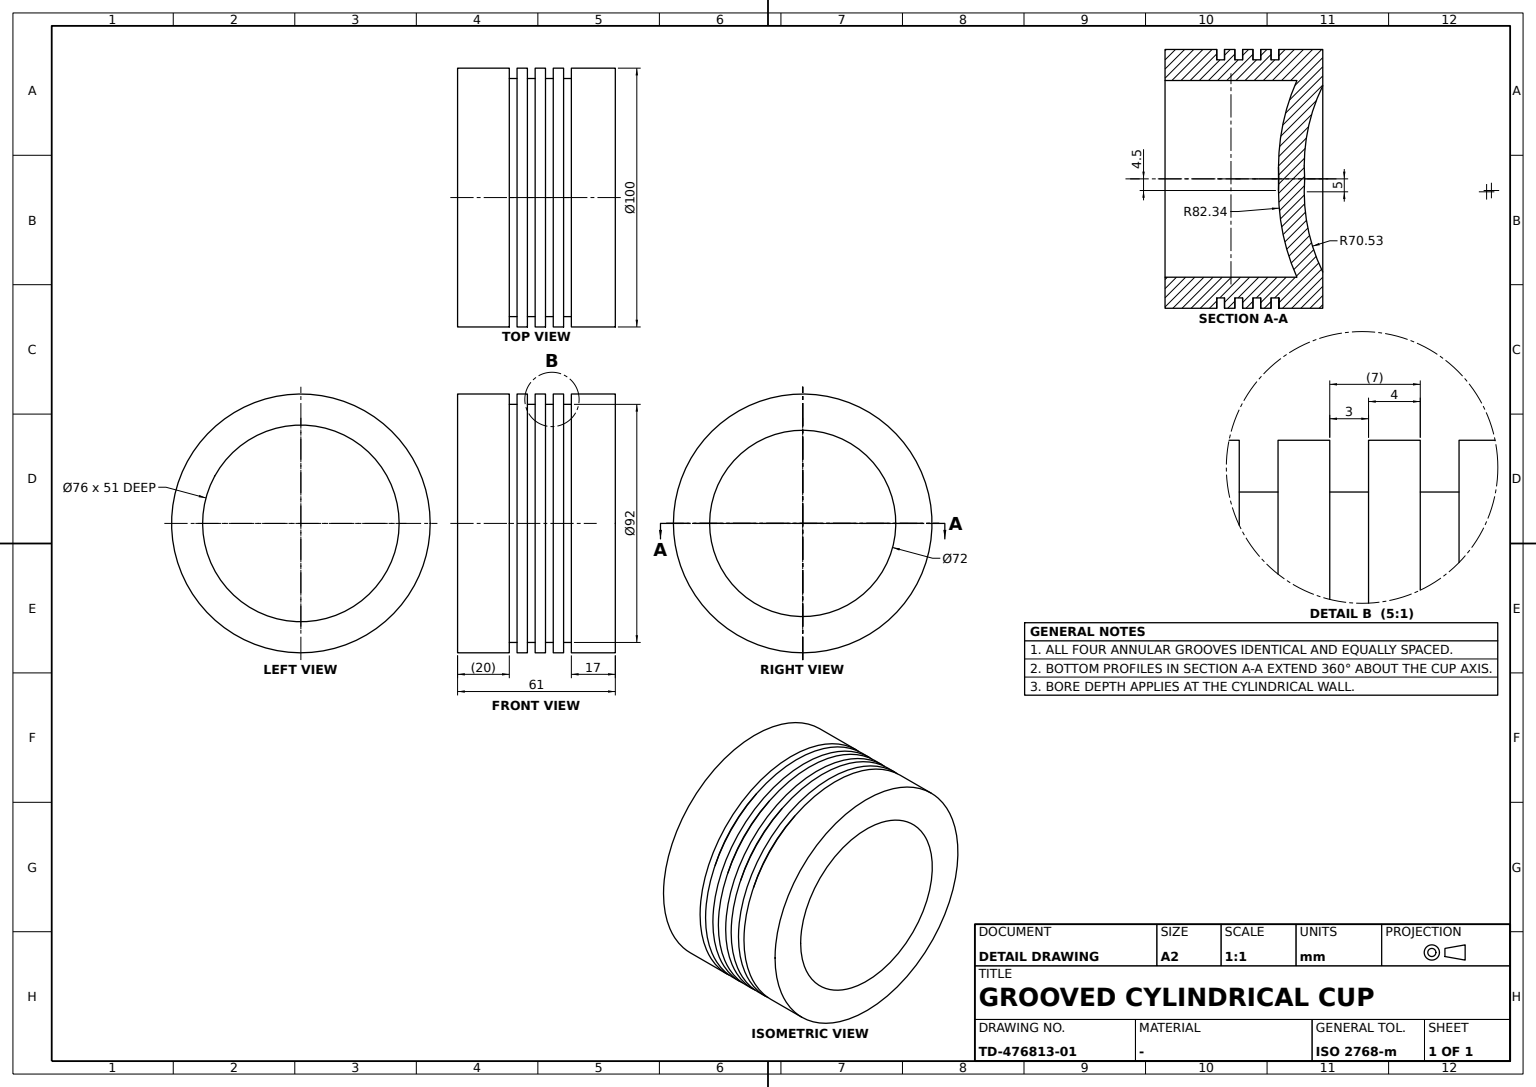
ISO-10303-21;
HEADER;
FILE_DESCRIPTION((''),'2;1');
FILE_NAME('','',(''),(''),'','','');
FILE_SCHEMA(('AUTOMOTIVE_DESIGN'));
ENDSEC;
DATA;
#1=APPLICATION_CONTEXT('');
#2=PRODUCT_CONTEXT('',#1,'mechanical');
#3=PRODUCT('','','',(#2));
#4=PRODUCT_DEFINITION_FORMATION('','',#3);
#5=PRODUCT_DEFINITION_CONTEXT('',#1,'design');
#6=PRODUCT_DEFINITION('','',#4,#5);
#7=PRODUCT_DEFINITION_SHAPE('','',#6);
#8=(LENGTH_UNIT()NAMED_UNIT(*)SI_UNIT(.MILLI.,.METRE.));
#9=(NAMED_UNIT(*)PLANE_ANGLE_UNIT()SI_UNIT($,.RADIAN.));
#10=(NAMED_UNIT(*)SI_UNIT($,.STERADIAN.)SOLID_ANGLE_UNIT());
#11=UNCERTAINTY_MEASURE_WITH_UNIT(LENGTH_MEASURE(1.E-05),#8,'distance_accuracy_value','');
#12=(GEOMETRIC_REPRESENTATION_CONTEXT(3)GLOBAL_UNCERTAINTY_ASSIGNED_CONTEXT((#11))GLOBAL_UNIT_ASSIGNED_CONTEXT((#8,#9,#10))REPRESENTATION_CONTEXT('',''));
#13=CARTESIAN_POINT('',(-40.368798,37.,22.053575));
#14=VERTEX_POINT('',#13);
#15=CARTESIAN_POINT('',(-40.368798,34.,22.053575));
#16=VERTEX_POINT('',#15);
#17=CARTESIAN_POINT('',(-40.368798,32.,22.053575));
#18=DIRECTION('',(0.,-1.,0.));
#19=VECTOR('',#18,1000.);
#20=LINE('',#17,#19);
#21=EDGE_CURVE('',#14,#16,#20,.T.);
#22=ORIENTED_EDGE('',*,*,#21,.F.);
#23=CARTESIAN_POINT('',(40.368798,37.,-22.053575));
#24=VERTEX_POINT('',#23);
#25=CARTESIAN_POINT('',(0.,37.,0.));
#26=DIRECTION('',(0.,1.,0.));
#27=DIRECTION('',(1.,0.,0.));
#28=AXIS2_PLACEMENT_3D('',#25,#26,#27);
#29=CIRCLE('',#28,46.);
#30=EDGE_CURVE('',#24,#14,#29,.T.);
#31=ORIENTED_EDGE('',*,*,#30,.F.);
#32=CARTESIAN_POINT('',(40.368798,34.,-22.053575));
#33=VERTEX_POINT('',#32);
#34=CARTESIAN_POINT('',(40.368798,32.,-22.053575));
#35=LINE('',#34,#19);
#36=EDGE_CURVE('',#24,#33,#35,.T.);
#37=ORIENTED_EDGE('',*,*,#36,.T.);
#38=CARTESIAN_POINT('',(0.,34.,0.));
#39=AXIS2_PLACEMENT_3D('',#38,#26,#27);
#40=CIRCLE('',#39,46.);
#41=EDGE_CURVE('',#33,#16,#40,.T.);
#42=ORIENTED_EDGE('',*,*,#41,.T.);
#43=EDGE_LOOP('',(#22,#31,#37,#42));
#44=FACE_OUTER_BOUND('',#43,.T.);
#45=CARTESIAN_POINT('',(0.,30.5,0.));
#46=AXIS2_PLACEMENT_3D('',#45,#18,#27);
#47=CYLINDRICAL_SURFACE('',#46,46.);
#48=ADVANCED_FACE('',(#44),#47,.T.);
#49=CARTESIAN_POINT('',(-43.879128,27.,23.971277));
#50=VERTEX_POINT('',#49);
#51=CARTESIAN_POINT('',(50.,27.,0.));
#52=VERTEX_POINT('',#51);
#53=CARTESIAN_POINT('',(0.,27.,0.));
#54=AXIS2_PLACEMENT_3D('',#53,#26,#27);
#55=CIRCLE('',#54,50.);
#56=EDGE_CURVE('',#50,#52,#55,.T.);
#57=ORIENTED_EDGE('',*,*,#56,.T.);
#58=CARTESIAN_POINT('',(43.879128,27.,-23.971277));
#59=VERTEX_POINT('',#58);
#60=EDGE_CURVE('',#52,#59,#55,.T.);
#61=ORIENTED_EDGE('',*,*,#60,.T.);
#62=EDGE_CURVE('',#59,#50,#55,.T.);
#63=ORIENTED_EDGE('',*,*,#62,.T.);
#64=EDGE_LOOP('',(#57,#61,#63));
#65=FACE_OUTER_BOUND('',#64,.T.);
#66=CARTESIAN_POINT('',(-40.368798,27.,22.053575));
#67=VERTEX_POINT('',#66);
#68=CARTESIAN_POINT('',(46.,27.,0.));
#69=VERTEX_POINT('',#68);
#70=CIRCLE('',#54,46.);
#71=EDGE_CURVE('',#67,#69,#70,.T.);
#72=ORIENTED_EDGE('',*,*,#71,.F.);
#73=CARTESIAN_POINT('',(40.368798,27.,-22.053575));
#74=VERTEX_POINT('',#73);
#75=EDGE_CURVE('',#74,#67,#70,.T.);
#76=ORIENTED_EDGE('',*,*,#75,.F.);
#77=EDGE_CURVE('',#69,#74,#70,.T.);
#78=ORIENTED_EDGE('',*,*,#77,.F.);
#79=EDGE_LOOP('',(#72,#76,#78));
#80=FACE_BOUND('',#79,.T.);
#81=CARTESIAN_POINT('',(-46.,27.,0.));
#82=AXIS2_PLACEMENT_3D('',#81,#26,#27);
#83=PLANE('',#82);
#84=ADVANCED_FACE('',(#65,#80),#83,.T.);
#85=ORIENTED_EDGE('',*,*,#75,.T.);
#86=CARTESIAN_POINT('',(-40.368798,30.,22.053575));
#87=VERTEX_POINT('',#86);
#88=EDGE_CURVE('',#87,#67,#20,.T.);
#89=ORIENTED_EDGE('',*,*,#88,.F.);
#90=CARTESIAN_POINT('',(40.368798,30.,-22.053575));
#91=VERTEX_POINT('',#90);
#92=CARTESIAN_POINT('',(0.,30.,0.));
#93=AXIS2_PLACEMENT_3D('',#92,#26,#27);
#94=CIRCLE('',#93,46.);
#95=EDGE_CURVE('',#91,#87,#94,.T.);
#96=ORIENTED_EDGE('',*,*,#95,.F.);
#97=EDGE_CURVE('',#91,#74,#35,.T.);
#98=ORIENTED_EDGE('',*,*,#97,.T.);
#99=EDGE_LOOP('',(#85,#89,#96,#98));
#100=FACE_OUTER_BOUND('',#99,.T.);
#101=ADVANCED_FACE('',(#100),#47,.T.);
#102=CARTESIAN_POINT('',(31.592972,61.,-17.259319));
#103=VERTEX_POINT('',#102);
#104=CARTESIAN_POINT('',(-31.592972,61.,17.259319));
#105=VERTEX_POINT('',#104);
#106=CARTESIAN_POINT('',(0.,61.,0.));
#107=AXIS2_PLACEMENT_3D('',#106,#26,#27);
#108=CIRCLE('',#107,36.);
#109=EDGE_CURVE('',#103,#105,#108,.T.);
#110=ORIENTED_EDGE('',*,*,#109,.T.);
#111=CARTESIAN_POINT('',(0.,54.,0.));
#112=VERTEX_POINT('',#111);
#113=CARTESIAN_POINT('',(-4.387913,124.357143,2.397128));
#114=DIRECTION('',(-0.479425539,0.,-0.877582562));
#115=DIRECTION('',(-0.877582562,0.,0.479425539));
#116=AXIS2_PLACEMENT_3D('',#113,#114,#115);
#117=CIRCLE('',#116,70.534584);
#118=EDGE_CURVE('',#112,#105,#117,.T.);
#119=ORIENTED_EDGE('',*,*,#118,.F.);
#120=CARTESIAN_POINT('',(4.387913,124.357143,-2.397128));
#121=DIRECTION('',(0.479425539,0.,0.877582562));
#122=DIRECTION('',(0.877582562,0.,-0.479425539));
#123=AXIS2_PLACEMENT_3D('',#120,#121,#122);
#124=CIRCLE('',#123,70.534584);
#125=EDGE_CURVE('',#112,#103,#124,.T.);
#126=ORIENTED_EDGE('',*,*,#125,.T.);
#127=EDGE_LOOP('',(#110,#119,#126));
#128=FACE_OUTER_BOUND('',#127,.T.);
#129=CARTESIAN_POINT('',(0.,124.357143,0.));
#130=AXIS2_PLACEMENT_3D('',#129,#26,#27);
#131=TOROIDAL_SURFACE('',#130,5.,70.534584);
#132=ADVANCED_FACE('',(#128),#131,.F.);
#133=CARTESIAN_POINT('',(-40.368798,44.,22.053575));
#134=VERTEX_POINT('',#133);
#135=CARTESIAN_POINT('',(46.,44.,0.));
#136=VERTEX_POINT('',#135);
#137=CARTESIAN_POINT('',(0.,44.,0.));
#138=AXIS2_PLACEMENT_3D('',#137,#26,#27);
#139=CIRCLE('',#138,46.);
#140=EDGE_CURVE('',#134,#136,#139,.T.);
#141=ORIENTED_EDGE('',*,*,#140,.F.);
#142=CARTESIAN_POINT('',(-40.368798,41.,22.053575));
#143=VERTEX_POINT('',#142);
#144=EDGE_CURVE('',#134,#143,#20,.T.);
#145=ORIENTED_EDGE('',*,*,#144,.T.);
#146=CARTESIAN_POINT('',(46.,41.,0.));
#147=VERTEX_POINT('',#146);
#148=CARTESIAN_POINT('',(0.,41.,0.));
#149=AXIS2_PLACEMENT_3D('',#148,#26,#27);
#150=CIRCLE('',#149,46.);
#151=EDGE_CURVE('',#143,#147,#150,.T.);
#152=ORIENTED_EDGE('',*,*,#151,.T.);
#153=CARTESIAN_POINT('',(46.,30.5,0.));
#154=LINE('',#153,#19);
#155=EDGE_CURVE('',#136,#147,#154,.T.);
#156=ORIENTED_EDGE('',*,*,#155,.F.);
#157=EDGE_LOOP('',(#141,#145,#152,#156));
#158=FACE_OUTER_BOUND('',#157,.T.);
#159=ADVANCED_FACE('',(#158),#47,.T.);
#160=CARTESIAN_POINT('',(43.879128,23.,-23.971277));
#161=VERTEX_POINT('',#160);
#162=CARTESIAN_POINT('',(-43.879128,23.,23.971277));
#163=VERTEX_POINT('',#162);
#164=CARTESIAN_POINT('',(0.,23.,0.));
#165=AXIS2_PLACEMENT_3D('',#164,#26,#27);
#166=CIRCLE('',#165,50.);
#167=EDGE_CURVE('',#161,#163,#166,.T.);
#168=ORIENTED_EDGE('',*,*,#167,.T.);
#169=CARTESIAN_POINT('',(-43.879128,30.5,23.971277));
#170=LINE('',#169,#19);
#171=EDGE_CURVE('',#50,#163,#170,.T.);
#172=ORIENTED_EDGE('',*,*,#171,.F.);
#173=ORIENTED_EDGE('',*,*,#62,.F.);
#174=CARTESIAN_POINT('',(43.879128,30.5,-23.971277));
#175=LINE('',#174,#19);
#176=EDGE_CURVE('',#59,#161,#175,.T.);
#177=ORIENTED_EDGE('',*,*,#176,.T.);
#178=EDGE_LOOP('',(#168,#172,#173,#177));
#179=FACE_OUTER_BOUND('',#178,.T.);
#180=CYLINDRICAL_SURFACE('',#46,50.);
#181=ADVANCED_FACE('',(#179),#180,.T.);
#182=CARTESIAN_POINT('',(46.,37.,0.));
#183=VERTEX_POINT('',#182);
#184=EDGE_CURVE('',#14,#183,#29,.T.);
#185=ORIENTED_EDGE('',*,*,#184,.T.);
#186=EDGE_CURVE('',#183,#24,#29,.T.);
#187=ORIENTED_EDGE('',*,*,#186,.T.);
#188=ORIENTED_EDGE('',*,*,#30,.T.);
#189=EDGE_LOOP('',(#185,#187,#188));
#190=FACE_BOUND('',#189,.T.);
#191=CARTESIAN_POINT('',(50.,37.,0.));
#192=VERTEX_POINT('',#191);
#193=CARTESIAN_POINT('',(43.879128,37.,-23.971277));
#194=VERTEX_POINT('',#193);
#195=CIRCLE('',#28,50.);
#196=EDGE_CURVE('',#192,#194,#195,.T.);
#197=ORIENTED_EDGE('',*,*,#196,.F.);
#198=CARTESIAN_POINT('',(-43.879128,37.,23.971277));
#199=VERTEX_POINT('',#198);
#200=EDGE_CURVE('',#199,#192,#195,.T.);
#201=ORIENTED_EDGE('',*,*,#200,.F.);
#202=EDGE_CURVE('',#194,#199,#195,.T.);
#203=ORIENTED_EDGE('',*,*,#202,.F.);
#204=EDGE_LOOP('',(#197,#201,#203));
#205=FACE_OUTER_BOUND('',#204,.T.);
#206=CARTESIAN_POINT('',(-50.,37.,0.));
#207=AXIS2_PLACEMENT_3D('',#206,#26,#27);
#208=PLANE('',#207);
#209=ADVANCED_FACE('',(#190,#205),#208,.F.);
#210=CARTESIAN_POINT('',(46.,34.,0.));
#211=VERTEX_POINT('',#210);
#212=EDGE_CURVE('',#183,#211,#154,.T.);
#213=ORIENTED_EDGE('',*,*,#212,.T.);
#214=EDGE_CURVE('',#211,#33,#40,.T.);
#215=ORIENTED_EDGE('',*,*,#214,.T.);
#216=ORIENTED_EDGE('',*,*,#36,.F.);
#217=ORIENTED_EDGE('',*,*,#186,.F.);
#218=EDGE_LOOP('',(#213,#215,#216,#217));
#219=FACE_OUTER_BOUND('',#218,.T.);
#220=ADVANCED_FACE('',(#219),#47,.T.);
#221=CARTESIAN_POINT('',(43.879128,44.,-23.971277));
#222=VERTEX_POINT('',#221);
#223=CARTESIAN_POINT('',(-43.879128,44.,23.971277));
#224=VERTEX_POINT('',#223);
#225=CIRCLE('',#138,50.);
#226=EDGE_CURVE('',#222,#224,#225,.T.);
#227=ORIENTED_EDGE('',*,*,#226,.T.);
#228=CARTESIAN_POINT('',(-43.879128,61.,23.971277));
#229=VERTEX_POINT('',#228);
#230=EDGE_CURVE('',#229,#224,#170,.T.);
#231=ORIENTED_EDGE('',*,*,#230,.F.);
#232=CARTESIAN_POINT('',(43.879128,61.,-23.971277));
#233=VERTEX_POINT('',#232);
#234=CIRCLE('',#107,50.);
#235=EDGE_CURVE('',#233,#229,#234,.T.);
#236=ORIENTED_EDGE('',*,*,#235,.F.);
#237=EDGE_CURVE('',#233,#222,#175,.T.);
#238=ORIENTED_EDGE('',*,*,#237,.T.);
#239=EDGE_LOOP('',(#227,#231,#236,#238));
#240=FACE_OUTER_BOUND('',#239,.T.);
#241=ADVANCED_FACE('',(#240),#180,.T.);
#242=CARTESIAN_POINT('',(40.368798,41.,-22.053575));
#243=VERTEX_POINT('',#242);
#244=EDGE_CURVE('',#147,#243,#150,.T.);
#245=ORIENTED_EDGE('',*,*,#244,.F.);
#246=ORIENTED_EDGE('',*,*,#151,.F.);
#247=EDGE_CURVE('',#243,#143,#150,.T.);
#248=ORIENTED_EDGE('',*,*,#247,.F.);
#249=EDGE_LOOP('',(#245,#246,#248));
#250=FACE_BOUND('',#249,.T.);
#251=CARTESIAN_POINT('',(-43.879128,41.,23.971277));
#252=VERTEX_POINT('',#251);
#253=CARTESIAN_POINT('',(50.,41.,0.));
#254=VERTEX_POINT('',#253);
#255=CIRCLE('',#149,50.);
#256=EDGE_CURVE('',#252,#254,#255,.T.);
#257=ORIENTED_EDGE('',*,*,#256,.T.);
#258=CARTESIAN_POINT('',(43.879128,41.,-23.971277));
#259=VERTEX_POINT('',#258);
#260=EDGE_CURVE('',#254,#259,#255,.T.);
#261=ORIENTED_EDGE('',*,*,#260,.T.);
#262=EDGE_CURVE('',#259,#252,#255,.T.);
#263=ORIENTED_EDGE('',*,*,#262,.T.);
#264=EDGE_LOOP('',(#257,#261,#263));
#265=FACE_OUTER_BOUND('',#264,.T.);
#266=CARTESIAN_POINT('',(-46.,41.,0.));
#267=AXIS2_PLACEMENT_3D('',#266,#26,#27);
#268=PLANE('',#267);
#269=ADVANCED_FACE('',(#250,#265),#268,.T.);
#270=CARTESIAN_POINT('',(46.,30.,0.));
#271=VERTEX_POINT('',#270);
#272=EDGE_CURVE('',#271,#69,#154,.T.);
#273=ORIENTED_EDGE('',*,*,#272,.F.);
#274=EDGE_CURVE('',#87,#271,#94,.T.);
#275=ORIENTED_EDGE('',*,*,#274,.F.);
#276=ORIENTED_EDGE('',*,*,#88,.T.);
#277=ORIENTED_EDGE('',*,*,#71,.T.);
#278=EDGE_LOOP('',(#273,#275,#276,#277));
#279=FACE_OUTER_BOUND('',#278,.T.);
#280=ADVANCED_FACE('',(#279),#47,.T.);
#281=ORIENTED_EDGE('',*,*,#97,.F.);
#282=EDGE_CURVE('',#271,#91,#94,.T.);
#283=ORIENTED_EDGE('',*,*,#282,.F.);
#284=ORIENTED_EDGE('',*,*,#272,.T.);
#285=ORIENTED_EDGE('',*,*,#77,.T.);
#286=EDGE_LOOP('',(#281,#283,#284,#285));
#287=FACE_OUTER_BOUND('',#286,.T.);
#288=ADVANCED_FACE('',(#287),#47,.T.);
#289=CARTESIAN_POINT('',(40.368798,44.,-22.053575));
#290=VERTEX_POINT('',#289);
#291=EDGE_CURVE('',#290,#243,#35,.T.);
#292=ORIENTED_EDGE('',*,*,#291,.T.);
#293=ORIENTED_EDGE('',*,*,#247,.T.);
#294=ORIENTED_EDGE('',*,*,#144,.F.);
#295=EDGE_CURVE('',#290,#134,#139,.T.);
#296=ORIENTED_EDGE('',*,*,#295,.F.);
#297=EDGE_LOOP('',(#292,#293,#294,#296));
#298=FACE_OUTER_BOUND('',#297,.T.);
#299=ADVANCED_FACE('',(#298),#47,.T.);
#300=CARTESIAN_POINT('',(-33.348137,0.,18.21817));
#301=VERTEX_POINT('',#300);
#302=CARTESIAN_POINT('',(-33.348137,51.,18.21817));
#303=VERTEX_POINT('',#302);
#304=CARTESIAN_POINT('',(-33.348137,25.5,18.21817));
#305=VECTOR('',#26,1000.);
#306=LINE('',#304,#305);
#307=EDGE_CURVE('',#301,#303,#306,.T.);
#308=ORIENTED_EDGE('',*,*,#307,.T.);
#309=CARTESIAN_POINT('',(38.,51.,0.));
#310=VERTEX_POINT('',#309);
#311=CARTESIAN_POINT('',(0.,51.,0.));
#312=AXIS2_PLACEMENT_3D('',#311,#26,#27);
#313=CIRCLE('',#312,38.);
#314=EDGE_CURVE('',#303,#310,#313,.T.);
#315=ORIENTED_EDGE('',*,*,#314,.T.);
#316=CARTESIAN_POINT('',(38.,0.,0.));
#317=VERTEX_POINT('',#316);
#318=CARTESIAN_POINT('',(38.,30.5,0.));
#319=LINE('',#318,#19);
#320=EDGE_CURVE('',#310,#317,#319,.T.);
#321=ORIENTED_EDGE('',*,*,#320,.T.);
#322=CARTESIAN_POINT('',(0.,0.,0.));
#323=AXIS2_PLACEMENT_3D('',#322,#26,#27);
#324=CIRCLE('',#323,38.);
#325=EDGE_CURVE('',#301,#317,#324,.T.);
#326=ORIENTED_EDGE('',*,*,#325,.F.);
#327=EDGE_LOOP('',(#308,#315,#321,#326));
#328=FACE_OUTER_BOUND('',#327,.T.);
#329=CYLINDRICAL_SURFACE('',#46,38.);
#330=ADVANCED_FACE('',(#328),#329,.F.);
#331=CARTESIAN_POINT('',(36.,61.,0.));
#332=VERTEX_POINT('',#331);
#333=EDGE_CURVE('',#105,#332,#108,.T.);
#334=ORIENTED_EDGE('',*,*,#333,.F.);
#335=ORIENTED_EDGE('',*,*,#109,.F.);
#336=EDGE_CURVE('',#332,#103,#108,.T.);
#337=ORIENTED_EDGE('',*,*,#336,.F.);
#338=EDGE_LOOP('',(#334,#335,#337));
#339=FACE_BOUND('',#338,.T.);
#340=ORIENTED_EDGE('',*,*,#235,.T.);
#341=CARTESIAN_POINT('',(50.,61.,0.));
#342=VERTEX_POINT('',#341);
#343=EDGE_CURVE('',#229,#342,#234,.T.);
#344=ORIENTED_EDGE('',*,*,#343,.T.);
#345=EDGE_CURVE('',#342,#233,#234,.T.);
#346=ORIENTED_EDGE('',*,*,#345,.T.);
#347=EDGE_LOOP('',(#340,#344,#346));
#348=FACE_OUTER_BOUND('',#347,.T.);
#349=CARTESIAN_POINT('',(-36.,61.,0.));
#350=AXIS2_PLACEMENT_3D('',#349,#26,#27);
#351=PLANE('',#350);
#352=ADVANCED_FACE('',(#339,#348),#351,.T.);
#353=CARTESIAN_POINT('',(40.368798,23.,-22.053575));
#354=VERTEX_POINT('',#353);
#355=CARTESIAN_POINT('',(40.368798,20.,-22.053575));
#356=VERTEX_POINT('',#355);
#357=EDGE_CURVE('',#354,#356,#35,.T.);
#358=ORIENTED_EDGE('',*,*,#357,.T.);
#359=CARTESIAN_POINT('',(-40.368798,20.,22.053575));
#360=VERTEX_POINT('',#359);
#361=CARTESIAN_POINT('',(0.,20.,0.));
#362=AXIS2_PLACEMENT_3D('',#361,#26,#27);
#363=CIRCLE('',#362,46.);
#364=EDGE_CURVE('',#356,#360,#363,.T.);
#365=ORIENTED_EDGE('',*,*,#364,.T.);
#366=CARTESIAN_POINT('',(-40.368798,23.,22.053575));
#367=VERTEX_POINT('',#366);
#368=EDGE_CURVE('',#367,#360,#20,.T.);
#369=ORIENTED_EDGE('',*,*,#368,.F.);
#370=CIRCLE('',#165,46.);
#371=EDGE_CURVE('',#354,#367,#370,.T.);
#372=ORIENTED_EDGE('',*,*,#371,.F.);
#373=EDGE_LOOP('',(#358,#365,#369,#372));
#374=FACE_OUTER_BOUND('',#373,.T.);
#375=ADVANCED_FACE('',(#374),#47,.T.);
#376=CARTESIAN_POINT('',(43.879128,20.,-23.971277));
#377=VERTEX_POINT('',#376);
#378=CARTESIAN_POINT('',(43.879128,0.,-23.971277));
#379=VERTEX_POINT('',#378);
#380=EDGE_CURVE('',#377,#379,#175,.T.);
#381=ORIENTED_EDGE('',*,*,#380,.T.);
#382=CARTESIAN_POINT('',(-43.879128,0.,23.971277));
#383=VERTEX_POINT('',#382);
#384=CIRCLE('',#323,50.);
#385=EDGE_CURVE('',#379,#383,#384,.T.);
#386=ORIENTED_EDGE('',*,*,#385,.T.);
#387=CARTESIAN_POINT('',(-43.879128,20.,23.971277));
#388=VERTEX_POINT('',#387);
#389=EDGE_CURVE('',#388,#383,#170,.T.);
#390=ORIENTED_EDGE('',*,*,#389,.F.);
#391=CIRCLE('',#362,50.);
#392=EDGE_CURVE('',#377,#388,#391,.T.);
#393=ORIENTED_EDGE('',*,*,#392,.F.);
#394=EDGE_LOOP('',(#381,#386,#390,#393));
#395=FACE_OUTER_BOUND('',#394,.T.);
#396=ADVANCED_FACE('',(#395),#180,.T.);
#397=EDGE_CURVE('',#136,#290,#139,.T.);
#398=ORIENTED_EDGE('',*,*,#397,.T.);
#399=ORIENTED_EDGE('',*,*,#295,.T.);
#400=ORIENTED_EDGE('',*,*,#140,.T.);
#401=EDGE_LOOP('',(#398,#399,#400));
#402=FACE_BOUND('',#401,.T.);
#403=CARTESIAN_POINT('',(50.,44.,0.));
#404=VERTEX_POINT('',#403);
#405=EDGE_CURVE('',#224,#404,#225,.T.);
#406=ORIENTED_EDGE('',*,*,#405,.F.);
#407=ORIENTED_EDGE('',*,*,#226,.F.);
#408=EDGE_CURVE('',#404,#222,#225,.T.);
#409=ORIENTED_EDGE('',*,*,#408,.F.);
#410=EDGE_LOOP('',(#406,#407,#409));
#411=FACE_OUTER_BOUND('',#410,.T.);
#412=CARTESIAN_POINT('',(-50.,44.,0.));
#413=AXIS2_PLACEMENT_3D('',#412,#26,#27);
#414=PLANE('',#413);
#415=ADVANCED_FACE('',(#402,#411),#414,.F.);
#416=CARTESIAN_POINT('',(46.,20.,0.));
#417=VERTEX_POINT('',#416);
#418=EDGE_CURVE('',#417,#356,#363,.T.);
#419=ORIENTED_EDGE('',*,*,#418,.F.);
#420=EDGE_CURVE('',#360,#417,#363,.T.);
#421=ORIENTED_EDGE('',*,*,#420,.F.);
#422=ORIENTED_EDGE('',*,*,#364,.F.);
#423=EDGE_LOOP('',(#419,#421,#422));
#424=FACE_BOUND('',#423,.T.);
#425=ORIENTED_EDGE('',*,*,#392,.T.);
#426=CARTESIAN_POINT('',(50.,20.,0.));
#427=VERTEX_POINT('',#426);
#428=EDGE_CURVE('',#388,#427,#391,.T.);
#429=ORIENTED_EDGE('',*,*,#428,.T.);
#430=EDGE_CURVE('',#427,#377,#391,.T.);
#431=ORIENTED_EDGE('',*,*,#430,.T.);
#432=EDGE_LOOP('',(#425,#429,#431));
#433=FACE_OUTER_BOUND('',#432,.T.);
#434=CARTESIAN_POINT('',(-46.,20.,0.));
#435=AXIS2_PLACEMENT_3D('',#434,#26,#27);
#436=PLANE('',#435);
#437=ADVANCED_FACE('',(#424,#433),#436,.T.);
#438=CARTESIAN_POINT('',(-43.879128,34.,23.971277));
#439=VERTEX_POINT('',#438);
#440=CARTESIAN_POINT('',(50.,34.,0.));
#441=VERTEX_POINT('',#440);
#442=CIRCLE('',#39,50.);
#443=EDGE_CURVE('',#439,#441,#442,.T.);
#444=ORIENTED_EDGE('',*,*,#443,.F.);
#445=CARTESIAN_POINT('',(-43.879128,30.,23.971277));
#446=VERTEX_POINT('',#445);
#447=EDGE_CURVE('',#439,#446,#170,.T.);
#448=ORIENTED_EDGE('',*,*,#447,.T.);
#449=CARTESIAN_POINT('',(50.,30.,0.));
#450=VERTEX_POINT('',#449);
#451=CIRCLE('',#93,50.);
#452=EDGE_CURVE('',#446,#450,#451,.T.);
#453=ORIENTED_EDGE('',*,*,#452,.T.);
#454=CARTESIAN_POINT('',(50.,30.5,0.));
#455=LINE('',#454,#19);
#456=EDGE_CURVE('',#441,#450,#455,.T.);
#457=ORIENTED_EDGE('',*,*,#456,.F.);
#458=EDGE_LOOP('',(#444,#448,#453,#457));
#459=FACE_OUTER_BOUND('',#458,.T.);
#460=ADVANCED_FACE('',(#459),#180,.T.);
#461=ORIENTED_EDGE('',*,*,#380,.F.);
#462=ORIENTED_EDGE('',*,*,#430,.F.);
#463=CARTESIAN_POINT('',(50.,0.,0.));
#464=VERTEX_POINT('',#463);
#465=EDGE_CURVE('',#427,#464,#455,.T.);
#466=ORIENTED_EDGE('',*,*,#465,.T.);
#467=EDGE_CURVE('',#464,#379,#384,.T.);
#468=ORIENTED_EDGE('',*,*,#467,.T.);
#469=EDGE_LOOP('',(#461,#462,#466,#468));
#470=FACE_OUTER_BOUND('',#469,.T.);
#471=ADVANCED_FACE('',(#470),#180,.T.);
#472=ORIENTED_EDGE('',*,*,#333,.T.);
#473=CARTESIAN_POINT('',(5.,124.357143,0.));
#474=DIRECTION('',(0.,0.,1.));
#475=AXIS2_PLACEMENT_3D('',#473,#474,#27);
#476=CIRCLE('',#475,70.534584);
#477=EDGE_CURVE('',#112,#332,#476,.T.);
#478=ORIENTED_EDGE('',*,*,#477,.F.);
#479=ORIENTED_EDGE('',*,*,#118,.T.);
#480=EDGE_LOOP('',(#472,#478,#479));
#481=FACE_OUTER_BOUND('',#480,.T.);
#482=ADVANCED_FACE('',(#481),#131,.F.);
#483=CARTESIAN_POINT('',(46.,23.,0.));
#484=VERTEX_POINT('',#483);
#485=EDGE_CURVE('',#484,#417,#154,.T.);
#486=ORIENTED_EDGE('',*,*,#485,.F.);
#487=EDGE_CURVE('',#367,#484,#370,.T.);
#488=ORIENTED_EDGE('',*,*,#487,.F.);
#489=ORIENTED_EDGE('',*,*,#368,.T.);
#490=ORIENTED_EDGE('',*,*,#420,.T.);
#491=EDGE_LOOP('',(#486,#488,#489,#490));
#492=FACE_OUTER_BOUND('',#491,.T.);
#493=ADVANCED_FACE('',(#492),#47,.T.);
#494=CARTESIAN_POINT('',(50.,23.,0.));
#495=VERTEX_POINT('',#494);
#496=EDGE_CURVE('',#52,#495,#455,.T.);
#497=ORIENTED_EDGE('',*,*,#496,.F.);
#498=ORIENTED_EDGE('',*,*,#56,.F.);
#499=ORIENTED_EDGE('',*,*,#171,.T.);
#500=EDGE_CURVE('',#163,#495,#166,.T.);
#501=ORIENTED_EDGE('',*,*,#500,.T.);
#502=EDGE_LOOP('',(#497,#498,#499,#501));
#503=FACE_OUTER_BOUND('',#502,.T.);
#504=ADVANCED_FACE('',(#503),#180,.T.);
#505=ORIENTED_EDGE('',*,*,#95,.T.);
#506=ORIENTED_EDGE('',*,*,#274,.T.);
#507=ORIENTED_EDGE('',*,*,#282,.T.);
#508=EDGE_LOOP('',(#505,#506,#507));
#509=FACE_BOUND('',#508,.T.);
#510=ORIENTED_EDGE('',*,*,#452,.F.);
#511=CARTESIAN_POINT('',(43.879128,30.,-23.971277));
#512=VERTEX_POINT('',#511);
#513=EDGE_CURVE('',#512,#446,#451,.T.);
#514=ORIENTED_EDGE('',*,*,#513,.F.);
#515=EDGE_CURVE('',#450,#512,#451,.T.);
#516=ORIENTED_EDGE('',*,*,#515,.F.);
#517=EDGE_LOOP('',(#510,#514,#516));
#518=FACE_OUTER_BOUND('',#517,.T.);
#519=CARTESIAN_POINT('',(-50.,30.,0.));
#520=AXIS2_PLACEMENT_3D('',#519,#26,#27);
#521=PLANE('',#520);
#522=ADVANCED_FACE('',(#509,#518),#521,.F.);
#523=ORIENTED_EDGE('',*,*,#320,.F.);
#524=CARTESIAN_POINT('',(33.348137,51.,-18.21817));
#525=VERTEX_POINT('',#524);
#526=EDGE_CURVE('',#310,#525,#313,.T.);
#527=ORIENTED_EDGE('',*,*,#526,.T.);
#528=CARTESIAN_POINT('',(33.348137,0.,-18.21817));
#529=VERTEX_POINT('',#528);
#530=CARTESIAN_POINT('',(33.348137,25.5,-18.21817));
#531=LINE('',#530,#305);
#532=EDGE_CURVE('',#529,#525,#531,.T.);
#533=ORIENTED_EDGE('',*,*,#532,.F.);
#534=EDGE_CURVE('',#317,#529,#324,.T.);
#535=ORIENTED_EDGE('',*,*,#534,.F.);
#536=EDGE_LOOP('',(#523,#527,#533,#535));
#537=FACE_OUTER_BOUND('',#536,.T.);
#538=ADVANCED_FACE('',(#537),#329,.F.);
#539=ORIENTED_EDGE('',*,*,#357,.F.);
#540=EDGE_CURVE('',#484,#354,#370,.T.);
#541=ORIENTED_EDGE('',*,*,#540,.F.);
#542=ORIENTED_EDGE('',*,*,#485,.T.);
#543=ORIENTED_EDGE('',*,*,#418,.T.);
#544=EDGE_LOOP('',(#539,#541,#542,#543));
#545=FACE_OUTER_BOUND('',#544,.T.);
#546=ADVANCED_FACE('',(#545),#47,.T.);
#547=ORIENTED_EDGE('',*,*,#202,.T.);
#548=EDGE_CURVE('',#252,#199,#170,.T.);
#549=ORIENTED_EDGE('',*,*,#548,.F.);
#550=ORIENTED_EDGE('',*,*,#262,.F.);
#551=EDGE_CURVE('',#259,#194,#175,.T.);
#552=ORIENTED_EDGE('',*,*,#551,.T.);
#553=EDGE_LOOP('',(#547,#549,#550,#552));
#554=FACE_OUTER_BOUND('',#553,.T.);
#555=ADVANCED_FACE('',(#554),#180,.T.);
#556=ORIENTED_EDGE('',*,*,#260,.F.);
#557=EDGE_CURVE('',#254,#192,#455,.T.);
#558=ORIENTED_EDGE('',*,*,#557,.T.);
#559=ORIENTED_EDGE('',*,*,#196,.T.);
#560=ORIENTED_EDGE('',*,*,#551,.F.);
#561=EDGE_LOOP('',(#556,#558,#559,#560));
#562=FACE_OUTER_BOUND('',#561,.T.);
#563=ADVANCED_FACE('',(#562),#180,.T.);
#564=ORIENTED_EDGE('',*,*,#343,.F.);
#565=ORIENTED_EDGE('',*,*,#230,.T.);
#566=ORIENTED_EDGE('',*,*,#405,.T.);
#567=EDGE_CURVE('',#342,#404,#455,.T.);
#568=ORIENTED_EDGE('',*,*,#567,.F.);
#569=EDGE_LOOP('',(#564,#565,#566,#568));
#570=FACE_OUTER_BOUND('',#569,.T.);
#571=ADVANCED_FACE('',(#570),#180,.T.);
#572=EDGE_CURVE('',#529,#301,#324,.T.);
#573=ORIENTED_EDGE('',*,*,#572,.F.);
#574=ORIENTED_EDGE('',*,*,#532,.T.);
#575=EDGE_CURVE('',#525,#303,#313,.T.);
#576=ORIENTED_EDGE('',*,*,#575,.T.);
#577=ORIENTED_EDGE('',*,*,#307,.F.);
#578=EDGE_LOOP('',(#573,#574,#576,#577));
#579=FACE_OUTER_BOUND('',#578,.T.);
#580=ADVANCED_FACE('',(#579),#329,.F.);
#581=ORIENTED_EDGE('',*,*,#200,.T.);
#582=ORIENTED_EDGE('',*,*,#557,.F.);
#583=ORIENTED_EDGE('',*,*,#256,.F.);
#584=ORIENTED_EDGE('',*,*,#548,.T.);
#585=EDGE_LOOP('',(#581,#582,#583,#584));
#586=FACE_OUTER_BOUND('',#585,.T.);
#587=ADVANCED_FACE('',(#586),#180,.T.);
#588=ORIENTED_EDGE('',*,*,#567,.T.);
#589=ORIENTED_EDGE('',*,*,#408,.T.);
#590=ORIENTED_EDGE('',*,*,#237,.F.);
#591=ORIENTED_EDGE('',*,*,#345,.F.);
#592=EDGE_LOOP('',(#588,#589,#590,#591));
#593=FACE_OUTER_BOUND('',#592,.T.);
#594=ADVANCED_FACE('',(#593),#180,.T.);
#595=ORIENTED_EDGE('',*,*,#184,.F.);
#596=ORIENTED_EDGE('',*,*,#21,.T.);
#597=EDGE_CURVE('',#16,#211,#40,.T.);
#598=ORIENTED_EDGE('',*,*,#597,.T.);
#599=ORIENTED_EDGE('',*,*,#212,.F.);
#600=EDGE_LOOP('',(#595,#596,#598,#599));
#601=FACE_OUTER_BOUND('',#600,.T.);
#602=ADVANCED_FACE('',(#601),#47,.T.);
#603=ORIENTED_EDGE('',*,*,#314,.F.);
#604=VERTEX_POINT('',#137);
#605=CARTESIAN_POINT('',(-3.949122,126.214286,2.157415));
#606=AXIS2_PLACEMENT_3D('',#605,#121,#115);
#607=CIRCLE('',#606,82.337347);
#608=EDGE_CURVE('',#303,#604,#607,.T.);
#609=ORIENTED_EDGE('',*,*,#608,.T.);
#610=CARTESIAN_POINT('',(4.5,126.214286,0.));
#611=AXIS2_PLACEMENT_3D('',#610,#474,#27);
#612=CIRCLE('',#611,82.337347);
#613=EDGE_CURVE('',#604,#310,#612,.T.);
#614=ORIENTED_EDGE('',*,*,#613,.T.);
#615=EDGE_LOOP('',(#603,#609,#614));
#616=FACE_OUTER_BOUND('',#615,.T.);
#617=CARTESIAN_POINT('',(0.,126.214286,0.));
#618=AXIS2_PLACEMENT_3D('',#617,#26,#27);
#619=TOROIDAL_SURFACE('',#618,4.5,82.337347);
#620=ADVANCED_FACE('',(#616),#619,.T.);
#621=ORIENTED_EDGE('',*,*,#389,.T.);
#622=EDGE_CURVE('',#383,#464,#384,.T.);
#623=ORIENTED_EDGE('',*,*,#622,.T.);
#624=ORIENTED_EDGE('',*,*,#465,.F.);
#625=ORIENTED_EDGE('',*,*,#428,.F.);
#626=EDGE_LOOP('',(#621,#623,#624,#625));
#627=FACE_OUTER_BOUND('',#626,.T.);
#628=ADVANCED_FACE('',(#627),#180,.T.);
#629=CARTESIAN_POINT('',(43.879128,34.,-23.971277));
#630=VERTEX_POINT('',#629);
#631=EDGE_CURVE('',#630,#439,#442,.T.);
#632=ORIENTED_EDGE('',*,*,#631,.T.);
#633=ORIENTED_EDGE('',*,*,#443,.T.);
#634=EDGE_CURVE('',#441,#630,#442,.T.);
#635=ORIENTED_EDGE('',*,*,#634,.T.);
#636=EDGE_LOOP('',(#632,#633,#635));
#637=FACE_OUTER_BOUND('',#636,.T.);
#638=ORIENTED_EDGE('',*,*,#41,.F.);
#639=ORIENTED_EDGE('',*,*,#214,.F.);
#640=ORIENTED_EDGE('',*,*,#597,.F.);
#641=EDGE_LOOP('',(#638,#639,#640));
#642=FACE_BOUND('',#641,.T.);
#643=CARTESIAN_POINT('',(-46.,34.,0.));
#644=AXIS2_PLACEMENT_3D('',#643,#26,#27);
#645=PLANE('',#644);
#646=ADVANCED_FACE('',(#637,#642),#645,.T.);
#647=EDGE_CURVE('',#630,#512,#175,.T.);
#648=ORIENTED_EDGE('',*,*,#647,.F.);
#649=ORIENTED_EDGE('',*,*,#634,.F.);
#650=ORIENTED_EDGE('',*,*,#456,.T.);
#651=ORIENTED_EDGE('',*,*,#515,.T.);
#652=EDGE_LOOP('',(#648,#649,#650,#651));
#653=FACE_OUTER_BOUND('',#652,.T.);
#654=ADVANCED_FACE('',(#653),#180,.T.);
#655=ORIENTED_EDGE('',*,*,#613,.F.);
#656=CARTESIAN_POINT('',(3.949122,126.214286,-2.157415));
#657=AXIS2_PLACEMENT_3D('',#656,#114,#122);
#658=CIRCLE('',#657,82.337347);
#659=EDGE_CURVE('',#525,#604,#658,.T.);
#660=ORIENTED_EDGE('',*,*,#659,.F.);
#661=ORIENTED_EDGE('',*,*,#526,.F.);
#662=EDGE_LOOP('',(#655,#660,#661));
#663=FACE_OUTER_BOUND('',#662,.T.);
#664=ADVANCED_FACE('',(#663),#619,.T.);
#665=ORIENTED_EDGE('',*,*,#496,.T.);
#666=EDGE_CURVE('',#495,#161,#166,.T.);
#667=ORIENTED_EDGE('',*,*,#666,.T.);
#668=ORIENTED_EDGE('',*,*,#176,.F.);
#669=ORIENTED_EDGE('',*,*,#60,.F.);
#670=EDGE_LOOP('',(#665,#667,#668,#669));
#671=FACE_OUTER_BOUND('',#670,.T.);
#672=ADVANCED_FACE('',(#671),#180,.T.);
#673=ORIENTED_EDGE('',*,*,#155,.T.);
#674=ORIENTED_EDGE('',*,*,#244,.T.);
#675=ORIENTED_EDGE('',*,*,#291,.F.);
#676=ORIENTED_EDGE('',*,*,#397,.F.);
#677=EDGE_LOOP('',(#673,#674,#675,#676));
#678=FACE_OUTER_BOUND('',#677,.T.);
#679=ADVANCED_FACE('',(#678),#47,.T.);
#680=ORIENTED_EDGE('',*,*,#622,.F.);
#681=ORIENTED_EDGE('',*,*,#385,.F.);
#682=ORIENTED_EDGE('',*,*,#467,.F.);
#683=EDGE_LOOP('',(#680,#681,#682));
#684=FACE_OUTER_BOUND('',#683,.T.);
#685=ORIENTED_EDGE('',*,*,#325,.T.);
#686=ORIENTED_EDGE('',*,*,#534,.T.);
#687=ORIENTED_EDGE('',*,*,#572,.T.);
#688=EDGE_LOOP('',(#685,#686,#687));
#689=FACE_BOUND('',#688,.T.);
#690=CARTESIAN_POINT('',(-50.,0.,0.));
#691=AXIS2_PLACEMENT_3D('',#690,#26,#27);
#692=PLANE('',#691);
#693=ADVANCED_FACE('',(#684,#689),#692,.F.);
#694=ORIENTED_EDGE('',*,*,#659,.T.);
#695=ORIENTED_EDGE('',*,*,#608,.F.);
#696=ORIENTED_EDGE('',*,*,#575,.F.);
#697=EDGE_LOOP('',(#694,#695,#696));
#698=FACE_OUTER_BOUND('',#697,.T.);
#699=ADVANCED_FACE('',(#698),#619,.T.);
#700=ORIENTED_EDGE('',*,*,#631,.F.);
#701=ORIENTED_EDGE('',*,*,#647,.T.);
#702=ORIENTED_EDGE('',*,*,#513,.T.);
#703=ORIENTED_EDGE('',*,*,#447,.F.);
#704=EDGE_LOOP('',(#700,#701,#702,#703));
#705=FACE_OUTER_BOUND('',#704,.T.);
#706=ADVANCED_FACE('',(#705),#180,.T.);
#707=ORIENTED_EDGE('',*,*,#167,.F.);
#708=ORIENTED_EDGE('',*,*,#666,.F.);
#709=ORIENTED_EDGE('',*,*,#500,.F.);
#710=EDGE_LOOP('',(#707,#708,#709));
#711=FACE_OUTER_BOUND('',#710,.T.);
#712=ORIENTED_EDGE('',*,*,#371,.T.);
#713=ORIENTED_EDGE('',*,*,#487,.T.);
#714=ORIENTED_EDGE('',*,*,#540,.T.);
#715=EDGE_LOOP('',(#712,#713,#714));
#716=FACE_BOUND('',#715,.T.);
#717=CARTESIAN_POINT('',(-50.,23.,0.));
#718=AXIS2_PLACEMENT_3D('',#717,#26,#27);
#719=PLANE('',#718);
#720=ADVANCED_FACE('',(#711,#716),#719,.F.);
#721=ORIENTED_EDGE('',*,*,#477,.T.);
#722=ORIENTED_EDGE('',*,*,#336,.T.);
#723=ORIENTED_EDGE('',*,*,#125,.F.);
#724=EDGE_LOOP('',(#721,#722,#723));
#725=FACE_OUTER_BOUND('',#724,.T.);
#726=ADVANCED_FACE('',(#725),#131,.F.);
#727=CLOSED_SHELL('',(#48,#84,#101,#132,#159,#181,#209,#220,#241,#269,#280,#288,#299,#330,#352,#375,#396,#415,#437,#460,#471,#482,#493,#504,#522,#538,#546,#555,#563,#571,#580,#587,#594,#602,#620,#628,#646,#654,#664,#672,#679,#693,#699,#706,#720,#726));
#728=MANIFOLD_SOLID_BREP('',#727);
#729=ADVANCED_BREP_SHAPE_REPRESENTATION('',(#728),#12);
#730=SHAPE_DEFINITION_REPRESENTATION(#7,#729);
ENDSEC;
END-ISO-10303-21;
